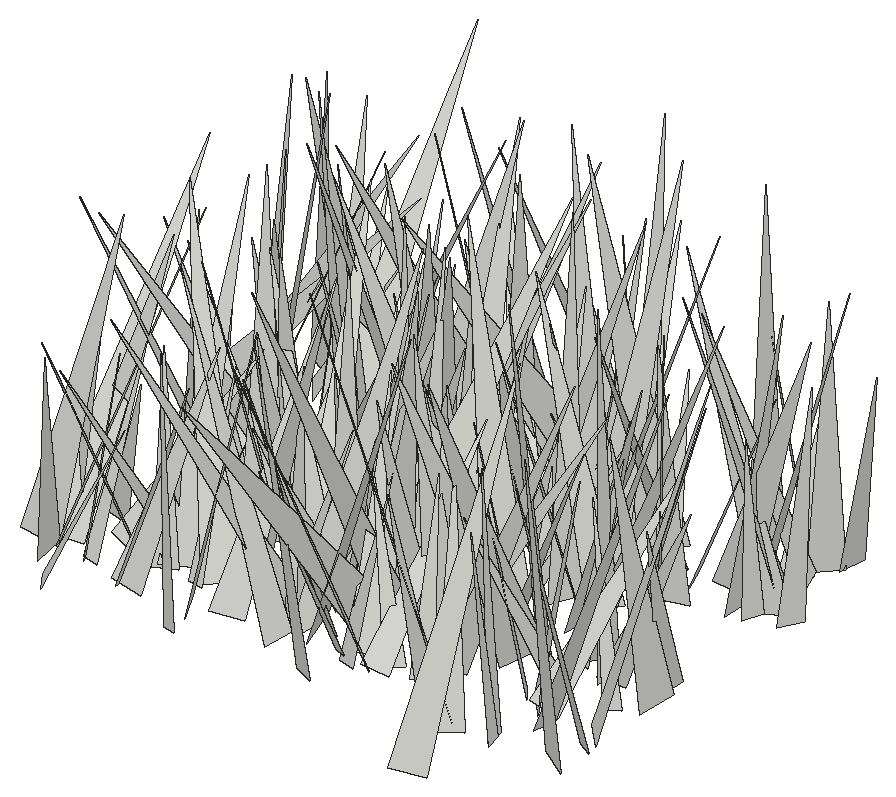
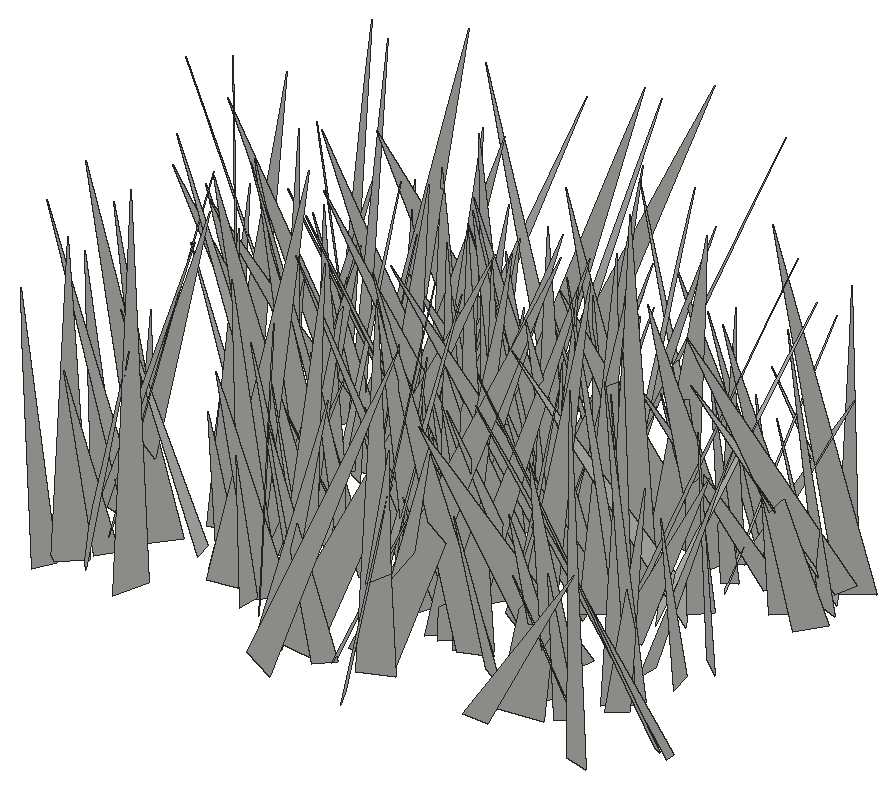
# SketchUp Ruby script. Lengths in inches.
U = 1.inch
M = Sketchup.active_model
def pt(a) = Geom::Point3d.new(a.map { |v| v * U })
def face(e, loops, mat)
  f = e.add_face(loops[0].map { |a| pt(a) })
  loops[1..].each { |l| e.add_face(l.map { |a| pt(a) }).erase! }
  f.material = f.back_material = mat if mat
  f
end
# faces: each face lists its corners as indices into pts; further lists are holes
def faces(e, pts, list, mat = nil) = list.each { |f| face(e, (f[0].is_a?(Array) ? f : [f]).map { |l| l.map { |i| pts[i] } }, mat) }
# xy, xz, yz: faces in a plane at the given z, y or x. An outline is a flat list of corners, or four numbers for a rectangle; further outlines are holes
def ring(l) = l.size == 4 ? [[l[0], l[1]], [l[2], l[1]], [l[2], l[3]], [l[0], l[3]]] : l.each_slice(2).to_a
def flat(e, list, mat, &to3) = list.each { |f| face(e, (f[0].is_a?(Array) ? f : [f]).map { |l| ring(l).map { |u, v| to3.(u, v) } }, mat) }
def xy(e, z, list, mat = nil) = flat(e, list, mat) { |x, y| [x, y, z] }
def xz(e, y, list, mat = nil) = flat(e, list, mat) { |x, z| [x, y, z] }
def yz(e, x, list, mat = nil) = flat(e, list, mat) { |y, z| [x, y, z] }
def lines(e, pts, list) = list.each { |a, b| e.add_line(pt(pts[a]), pt(pts[b])) }
# prism: a flat outline (further loops are holes) pulled along v
def prism(e, loops, v, mat = nil)
  f = face(e, loops, mat); d = Geom::Vector3d.new(v.map { |x| x * U })
  f.pushpull(f.normal.samedirection?(d) ? d.length : -d.length)
end
def box(e, o, s, mat = nil) = prism(e, [[o, [o[0] + s[0], o[1], o[2]], [o[0] + s[0], o[1] + s[1], o[2]], [o[0], o[1] + s[1], o[2]]]], [0, 0, s[2]], mat)
def at(x, y, z, deg = 0) = Geom::Transformation.translation(pt([x, y, z])) * Geom::Transformation.rotation(ORIGIN, Z_AXIS, deg.degrees)
def axes(o, x, y, z) = Geom::Transformation.new([*x, 0, *y, 0, *z, 0, *pt(o).to_a, 1])
def part(name) = M.definitions.add(name)
# library, detail: a bought-in or finely detailed component or shape, given as its bounding box
def library(name, o, s) = part(name).tap { |d| box(d.entities, o, s) }
def detail(e, o, s) = box(e.add_group.entities, o, s)
def put(e, d, t, mat = nil) = e.add_instance(d, t).tap { |i| i.material = mat if mat }
def group(e, t, mat = nil) = e.add_group.tap { |g| g.transformation = t; g.material = mat if mat }.entities
root = M.entities
c1 = part("fur_instance\#9")
p = [[0.8125,0,1.79],[0.67,-0.02,1.48],[0,-0.11,0],[0,0.11,0]]
faces(c1.entities,p,[[0,1,2,3]])
put(root,c1,axes([148.02,329.95,-27.1],[5.96387,-5.74764,0.45925],[-4.68382,-5.21453,-4.43673],[-3.36276,-2.93042,6.99418]))
put(root,c1,axes([148.79,327.89,-27.1],[-4.50054,-5.78959,0.45114],[-5.68851,4.51005,1.13049],[1.1678,-0.3432,7.24542]))
put(root,c1,axes([158.65,326.23,-27.1],[-3.10043,-5.65859,2.0595],[-5.81568,3.41455,0.62657],[1.56175,1.48157,6.42182]))
put(root,c1,axes([135.31,326.98,-27.1],[5.21183,-0.69159,1.00189],[-0.40075,-5.13378,-1.45906],[-1.14955,-1.3458,5.051]))
put(root,c1,axes([136.49,325.125,-27.1],[3.11612,2.14822,0.04863],[2.13222,-3.08072,-0.53874],[0.26618,-0.47091,3.74631]))
put(root,c1,axes([147.85,325.66,-27.1],[-3.61019,-4.99925,2.09321],[-5.40705,3.49453,-0.97958],[0.37125,2.28107,6.08822]))
put(root,c1,axes([144.81,329.15,-27.1],[-6.99156,-3.62516,0.34789],[-3.32905,6.6672,2.57109],[1.47657,-2.13338,7.444]))
put(root,c1,axes([156.08,326.05,-27.1],[-3.70453,-1.18645,1.17686],[-1.32576,3.8289,-0.31316],[1.01735,0.66938,3.87726]))
put(root,c1,axes([155.12,322.41,-27.1],[-6.41092,4.00729,0.82453],[3.32918,6.00061,-3.27831],[2.37798,2.40258,6.81256]))
put(root,c1,axes([154.44,325.61,-27.1],[-3.13208,3.88614,1.48189],[4.03166,3.29255,-0.11327],[1.02167,-1.07935,4.98991]))
put(root,c1,axes([142.17,325.18,-27.1],[2.11114,4.26728,1.69749],[4.08085,-2.60007,1.46097],[-2.10662,-0.76029,4.53125]))
put(root,c1,axes([152.23,327.2,-27.1],[0.17037,-4.40384,1.04145],[-4.5148,-0.2364,-0.26107],[-0.30825,1.02847,4.3994]))
put(root,c1,axes([153.88,326.43,-27.1],[-6.31099,-5.2237,1.0112],[-5.28027,5.95593,-2.18722],[-0.65451,2.31907,7.89505]))
put(root,c1,axes([141.64,327,-27.1],[5.91305,2.63208,1.30513],[2.84881,-5.85376,-1.10147],[-0.71801,-1.54954,6.37799]))
put(root,c1,axes([155.93,326.29,-27.1],[-4.75488,-0.89522,1.48594],[-1.16705,4.85843,-0.80746],[1.28353,1.10117,4.77057]))
put(root,c1,axes([147.875,327.68,-27.1],[-2.11494,-3.26023,0.3236],[-3.25153,2.04149,-0.68318],[-0.40176,0.64034,3.82562]))
put(root,c1,axes([138.71,326.98,-27.1],[4.6292,0.17151,0.50537],[0.17521,-4.6565,-0.02456],[-0.5041,-0.0434,4.63231]))
put(root,c1,axes([139.07,326.66,-27.1],[-0.2633,5.21725,2.01289],[5.21535,0.95622,-1.79623],[2.01778,-1.79073,4.90536]))
put(root,c1,axes([158.91,327.67,-27.1],[-3.27995,-3.84872,1.10692],[-4.00472,3.15616,-0.89264],[0.01123,1.42196,4.97734]))
put(root,c1,axes([146.15,328.58,-27.1],[7.97506,1.59703,0.67128],[1.71117,-7.75527,-1.87893],[-0.27022,-1.97686,7.91339]))
put(root,c1,axes([145.59,327.06,-27.1],[-7.05219,-0.0174,0.36445],[-0.04272,7.04446,-0.49029],[0.36236,0.49184,7.03515]))
put(root,c1,axes([138.22,330.29,-27.1],[-4.13321,-3.41194,0.20507],[-3.07913,3.85633,2.10107],[1.48403,-1.5014,4.93054]))
put(root,c1,axes([148.3125,330.61,-27.1],[0.33917,-8.30019,0.61155],[-8.21231,-0.43312,-1.32383],[-1.35096,0.54903,8.20095]))
put(root,c1,axes([138.89,328.01,-27.1],[-3.23089,-3.2407,0.20186],[-3.09319,2.98531,-1.58167],[-0.98745,1.25194,4.29408]))
put(root,c1,axes([134.44,327.56,-27.1],[1.86303,-6.4471,2.90273],[-6.99316,-1.23765,1.73947],[1.04242,3.21946,6.48153]))
put(root,c1,axes([146.71,328.67,-27.1],[-2.94659,-4.28728,0.79485],[-4.35538,2.84813,-0.78348],[-0.2081,1.09651,5.14289]))
put(root,c1,axes([153.12,331.42,-27.1],[6.488,-4.94571,0.82766],[-4.48999,-6.33233,-2.64212],[-2.23271,-1.63731,7.71838]))
put(root,c1,axes([150.02,328.08,-27.1],[-1.79664,3.17113,0.9039],[3.29721,1.71578,0.53432],[-0.03822,-1.04932,3.60534]))
put(root,c1,axes([136.61,327.37,-27.1],[2.93854,2.24557,1.05284],[2.03507,-3.11619,0.96641],[-1.41759,0.18132,3.56983]))
put(root,c1,axes([155.54,329.18,-27.1],[4.29125,3.34973,1.68987],[3.74545,-3.97458,-1.63261],[-0.21889,-2.33948,5.19327]))
put(root,c1,axes([145.97,328.53,-27.1],[-4.77809,0.40303,0.49366],[0.4272,4.79644,0.21897],[0.47289,-0.2608,4.79006]))
put(root,c1,axes([145.02,328.125,-27.1],[2.48119,3.58815,0.88423],[3.68479,-2.32113,-0.92071],[0.2811,-1.24521,4.2642]))
put(root,c1,axes([151.32,327.98,-27.1],[-2.54986,2.80817,1.27437],[2.87177,2.76487,-0.34653],[1.12374,-0.69377,3.77724]))
put(root,c1,axes([146.04,330.48,-27.1],[2.95419,-3.46444,1.08183],[-2.95275,-3.10527,-1.88109],[-2.11044,-0.50488,4.14621]))
put(root,c1,axes([139.31,328.55,-27.1],[1.67153,-3.68103,1.97281],[-4.08391,-1.88531,-0.05752],[-0.87388,1.76964,4.04237]))
put(root,c1,axes([136.89,327.36,-27.1],[1.45638,3.8911,0.37542],[3.87774,-1.48869,0.38679],[-0.49475,-0.21394,4.13668]))
put(root,c1,axes([154.88,330.97,-27.1],[-4.05266,-1.43323,0.72397],[-1.06557,3.87082,1.69814],[1.20119,-1.40176,3.94899]))
put(root,c1,axes([154.86,329.47,-27.1],[-3.48684,-2.54111,1.02639],[-2.66037,3.53733,-0.28017],[0.65812,0.83597,4.30544]))
put(root,c1,axes([134.55,329.12,-27.1],[2.41252,4.65389,1.89869],[5.02303,-2.30836,-0.72433],[-0.1815,-2.02404,5.19175]))
put(root,c1,axes([138.44,329.71,-27.1],[0.50859,-3.54434,0.97529],[-3.61365,-0.30136,0.78924],[0.67458,1.05784,3.49258]))
put(root,c1,axes([148.54,328.14,-27.1],[-2.22109,4.73282,1.14399],[4.81333,2.32397,-0.26934],[0.73496,-0.91711,5.22114]))
put(root,c1,axes([150.7,330.1875,-27.1],[3.54462,-5.56954,2.15269],[-5.7416,-3.86654,-0.54956],[-1.63946,1.49942,6.57891]))
put(root,c1,axes([135.71,330.37,-27.1],[0.50493,-3.90237,0.56248],[-3.75126,-0.30094,1.27958],[1.21364,0.69337,3.72104]))
put(root,c1,axes([149.64,327.45,-27.1],[-1.38897,4.86037,0.26759],[4.61521,1.40338,-1.53442],[1.54748,0.17706,4.81643]))
put(root,c1,axes([142.125,329.85,-27.1],[6.74375,-1.56753,0.95704],[-1.61805,-6.79399,0.27364],[-0.86892,0.48558,6.91813]))
put(root,c1,axes([140.84,328.32,-27.1],[1.32341,3.79294,0.4756],[3.74321,-1.38791,0.65276],[-0.77522,-0.22654,3.9638]))
put(root,c1,axes([142.03,331.95,-27.1],[-4.79038,-5.44103,1.36632],[-5.2062,4.98101,1.5825],[2.08977,-0.06337,7.07448]))
put(root,c1,axes([151.85,328.84,-27.1],[6.12264,-2.56902,1.18593],[-2.80714,-5.86992,1.77677],[-0.35534,2.10644,6.39763]))
put(root,c1,axes([151.7,332.15,-27.1],[4.33462,-5.23656,1.50263],[-4.77333,-4.57611,-2.17783],[-2.62578,-0.3257,6.43953]))
put(root,c1,axes([156.78,328.09,-27.1],[6.71372,1.26121,1.18447],[0.98901,-6.69183,1.51954],[-1.41968,1.3025,6.66001]))
put(root,c1,axes([148.57,327.17,-27.1],[3.46655,5.88623,0.70358],[5.62008,-3.5225,1.77941],[-1.8861,0.32244,6.59533]))
put(root,c1,axes([144,329.98,-27.1],[0.99186,4.25892,2.03749],[4.71935,-0.95274,-0.30591],[-0.13232,-2.05608,4.36218]))
put(root,c1,axes([141.59,329.05,-27.1],[-4.74257,5.72398,1.5327],[5.90767,4.72004,0.65254],[0.46105,-1.60076,7.40474]))
put(root,c1,axes([158.94,331.71,-27.1],[5.89812,-2.41371,1.85981],[-1.99813,-6.12286,-1.60962],[-2.30052,-0.87028,6.16628]))
put(root,c1,axes([158.6,328.57,-27.1],[5.3088,5.05785,1.00754],[5.10033,-5.36326,0.04959],[-0.76398,-0.65873,7.33231]))
put(root,c1,axes([143.11,327.25,-27.1],[-4.70627,4.28235,1.06672],[3.70191,4.67966,-2.45399],[2.40255,1.178,5.87073]))
put(root,c1,axes([148.3,331.74,-27.1],[-4.48343,0.78051,2.64752],[1.64873,4.80743,1.37477],[2.21365,-1.99978,4.33824]))
put(root,c1,axes([153.71,331.91,-27.1],[-3.953,-6.85404,2.35159],[-6.87911,4.39144,1.23577],[2.27722,1.36799,7.81517]))
put(root,c1,axes([136.97,329.07,-27.1],[0.32449,4.79651,0.65441],[4.29347,0.01783,-2.25961],[2.23626,-0.73022,4.24334]))
put(root,c1,axes([156.02,328.96,-27.1],[-0.77489,5.32124,0.74593],[4.8544,1.01638,-2.20776],[2.30365,-0.35187,4.90325]))
put(root,c1,axes([137.87,332.07,-27.1],[2.72527,-3.47225,0.02549],[-3.46346,-2.7159,0.33551],[0.24824,0.22715,4.40125]))
put(root,c1,axes([144.92,331.54,-27.1],[3.71508,-1.29272,0.27873],[-1.28155,-3.72443,-0.19222],[-0.32626,-0.0905,3.92887]))
put(root,c1,axes([134.17,330.49,-27.1],[3.16186,-4.77933,2.12939],[-5.21892,-2.70344,1.68164],[0.37303,2.68757,5.47827]))
put(root,c1,axes([135.22,327.62,-27.1],[5.40862,3.75774,0.29196],[3.28966,-4.95573,2.84217],[-1.83956,2.18614,5.94103]))
put(root,c1,axes([158.61,332.875,-27.1],[4.29129,-1.7599,0.57931],[-1.53313,-4.1935,-1.38278],[-1.04037,-1.07949,4.42723]))
put(root,c1,axes([157.96,330.41,-27.1],[-0.43735,3.78387,0.74816],[3.7266,0.2203,1.06426],[-0.99494,-0.83814,3.65736]))
put(root,c1,axes([145.99,332.95,-27.1],[2.29516,-7.21123,1.1617],[-7.23425,-2.07612,1.40519],[1.00849,1.5189,7.43607]))
put(root,c1,axes([139.01,333.09,-27.1],[-5.75391,-4.14909,0.07824],[-4.14913,5.75437,0.02082],[0.07564,0.02888,7.0938]))
put(root,c1,axes([156.68,331.96,-27.1],[2.75762,-4.13306,0.47465],[-3.98702,-2.46295,1.71739],[1.18791,1.32801,4.66232]))
put(root,c1,axes([139.53,328.97,-27.1],[-5.90287,3.96424,1.22936],[3.5461,5.92766,-2.08769],[2.15678,1.10365,6.7971]))
put(root,c1,axes([150.24,331.18,-27.1],[4.10846,4.74791,0.21399],[4.46685,-3.7608,-2.31765],[1.62348,-1.66782,5.83529]))
put(root,c1,axes([151.82,332.21,-27.1],[5.27208,0.02621,0.0042],[0.02652,-5.23568,-0.61848],[-0.0011,-0.61849,5.23574]))
put(root,c1,axes([135.03,328.06,-27.1],[-5.0261,5.87636,0.71878],[5.2638,4.86732,-2.98524],[2.70938,1.44485,7.13314]))
put(root,c1,axes([141.4,333.24,-27.1],[2.7716,-4.32676,0.73791],[-4.29866,-2.85215,-0.57784],[-0.88707,0.30254,5.10575]))
put(root,c1,axes([144.55,332.15,-27.1],[-1.98157,5.41612,3.08152],[6.10168,2.34277,-0.19399],[1.26474,-2.81671,5.76397]))
put(root,c1,axes([144.51,330.91,-27.1],[0.16131,6.95669,2.04491],[7.08472,0.28432,-1.5261],[1.54396,-2.03146,6.78915]))
put(root,c1,axes([146.39,331.33,-27.1],[-1.99924,6.11191,2.2816],[6.3463,2.375,-0.80119],[1.51181,-1.88733,6.38047]))
put(root,c1,axes([140.8,332.15,-27.1],[5.17413,-4.7343,3.23528],[-5.24163,-5.67192,0.08293],[-2.32507,2.25121,7.01272]))
put(root,c1,axes([143.2,332.24,-27.1],[-4.86777,3.35697,1.6535],[3.6105,4.92638,0.62739],[0.98366,-1.46972,5.8797]))
put(root,c1,axes([138.49,336.52,-27.1],[-6.95908,-3.88864,0.42907],[-3.38575,6.42493,3.31533],[1.96017,-2.70799,7.24975]))
put(root,c1,axes([156.37,332.2,-27.1],[-6.67663,-0.80436,2.4344],[-1.05353,7.05179,-0.55944],[2.33738,0.88086,6.7016]))
put(root,c1,axes([157.5,333.56,-27.1],[6.08028,3.66314,2.96745],[4.34842,-6.22849,-1.22118],[-1.82087,-2.64225,6.99265]))
put(root,c1,axes([140.65,334.31,-27.1],[4.51111,-4.76568,1.07484],[-4.75985,-4.61702,-0.49408],[-1.1004,0.43419,6.54353]))
put(root,c1,axes([154.84,332.49,-27.1],[2.00613,4.44684,1.43472],[4.67253,-1.91449,-0.59961],[-0.01581,-1.5549,4.84142]))
put(root,c1,axes([143.24,333.75,-27.1],[3.93197,-0.07434,1.3447],[0.21137,-4.06439,-0.84276],[-1.33006,-0.86567,3.84131]))
put(root,c1,axes([151.16,333.48,-27.1],[-2.98198,-2.20876,0.85448],[-2.34628,2.94214,-0.58291],[0.32208,0.98295,3.66484]))
put(root,c1,axes([153.21,334.51,-27.1],[6.29896,-1.22347,0.37639],[-1.1888,-6.29213,-0.55798],[-0.47466,-0.47719,6.39237]))
put(root,c1,axes([146.99,332.33,-27.1],[-6.72767,0.28008,1.7782],[-0.11729,6.79671,-1.51427],[1.7963,1.49276,6.56102]))
put(root,c1,axes([143.32,332.86,-27.1],[3.71678,-0.58843,1.31141],[-0.99782,-3.67326,1.17982],[-1.0346,1.42876,3.57333]))
put(root,c1,axes([151.24,336.56,-27.1],[-4.09949,-5.26965,1.04192],[-4.89422,4.20438,2.00758],[2.21389,-0.46331,6.36747]))
put(root,c1,axes([147.98,332.1,-27.1],[-6.09704,1.94582,1.05535],[1.61207,6.02238,-1.79053],[1.51697,1.42075,6.14444]))
put(root,c1,axes([147.14,334.9,-27.1],[-3.57828,-1.18752,0.86435],[-1.11493,3.67791,0.43741],[0.95617,-0.15551,3.74473]))
put(root,c1,axes([150.1,334.34,-27.1],[-5.03128,5.10175,2.45438],[5.52933,5.13327,0.66454],[1.21582,-2.23324,7.13442]))
put(root,c1,axes([155.03,332.48,-27.1],[6.92746,0.46404,1.30725],[0.06508,-6.75935,2.05449],[-1.38564,2.00246,6.63205]))
put(root,c1,axes([142.92,332.62,-27.1],[-3.90742,5.66938,0.63215],[5.60395,3.95813,-0.85923],[1.06639,-0.02677,6.83166]))
put(root,c1,axes([146.64,336.6,-27.1],[1.6071,-3.85332,0.26864],[-3.82652,-1.62792,-0.45895],[-0.52725,0.06941,4.14972]))
put(root,c1,axes([146.08,332.85,-27.1],[0.28527,8.21503,1.11931],[7.94931,0.04717,-2.37217],[2.35543,-1.15413,7.87026]))
put(root,c1,axes([146.5625,336.55,-27.1],[1.94153,-7.03493,2.68991],[-6.84514,-2.80689,-2.40016],[-3.14163,1.7682,6.89195]))
put(root,c1,axes([135.17,334.86,-27.1],[2.79154,3.79561,1.789],[3.98615,-3.06992,0.29332],[-1.31064,-1.25251,4.70248]))
put(root,c1,axes([138.73,335.11,-27.1],[-2.74524,3.88345,0.46197],[3.73915,2.44095,1.70042],[-1.14601,-1.33847,4.4414]))
put(root,c1,axes([149.73,335.05,-27.1],[1.87721,3.55983,2.07479],[3.45548,-2.60202,1.33802],[-2.2443,-1.02868,3.79553]))
put(root,c1,axes([155.05,335.29,-27.1],[4.65489,2.00226,0.76997],[2.06003,-4.68544,-0.26978],[-0.59848,-0.55448,5.06006]))
put(root,c1,axes([138.39,332.14,-27.1],[6.17595,4.1917,0.11311],[3.92557,-5.85042,2.46738],[-1.47413,1.98185,7.04448]))
put(root,c1,axes([145.65,335.82,-27.1],[-2.59622,-3.87524,1.56211],[-4.17566,2.47102,-0.8099],[0.14666,1.75346,4.59368]))
put(root,c1,axes([136.68,336.55,-27.1],[-4.93591,-0.64757,0.62999],[-0.58328,4.95621,0.52453],[0.68994,-0.44273,4.95049]))
put(root,c1,axes([142.77,335.02,-27.1],[4.39475,-2.24157,1.41228],[-2.61052,-4.13054,1.56743],[-0.4521,2.06082,4.67778]))
put(root,c1,axes([146.18,336.84,-27.1],[2.32734,-2.83374,0.7234],[-2.82694,-2.41664,-0.37171],[-0.74954,0.31569,3.64807]))
put(root,c1,axes([153.16,336.07,-27.1],[1.40362,-5.52471,3.15038],[-5.88186,-2.35471,-1.50878],[-2.41887,2.51999,5.49692]))
put(root,c1,axes([142.69,336.65,-27.1],[-2.18314,-4.32344,1.23175],[-4.48368,1.99494,-0.94459],[-0.32548,1.51774,4.75036]))
put(root,c1,axes([151.72,335.61,-27.1],[-6.82221,1.72842,2.33339],[1.55801,7.20655,-0.7829],[2.45045,0.23004,6.99407]))
put(root,c1,axes([150.13,336.11,-27.1],[2.36408,2.77163,0.06713],[2.67068,-2.25294,-1.03299],[0.74428,-0.71945,3.49339]))
put(root,c1,axes([143.6875,338.3,-27.1],[-2.92587,-7.18113,1.16279],[-7.26033,2.80394,-0.95233],[-0.45638,1.43204,7.69561]))
put(root,c1,axes([144.07,334.52,-27.1],[-6.55777,-1.69063,0.96933],[-1.94723,5.82112,-3.02077],[0.07829,3.17151,6.06115]))
put(root,c1,axes([143.35,338.85,-27.1],[6.03142,-3.81553,0.06105],[-3.78285,-5.99326,-0.84318],[-0.50203,-0.68018,7.08699]))
put(root,c1,axes([141.83,335.84,-27.1],[3.01287,6.59159,3.14785],[6.68601,-3.85992,1.68335],[-2.94198,-2.02171,7.04931]))
put(root,c1,axes([141.3,333.76,-27.1],[8.13391,1.72844,0.70897],[1.41113,-7.75982,2.72846],[-1.22428,2.53935,7.85515]))
put(root,c1,axes([144.98,334.99,-27.1],[4.52009,6.67395,0.30614],[6.59904,-4.40227,-1.46264],[1.04307,-1.07006,7.92676]))
put(root,c1,axes([142.47,339.125,-27.1],[1.32188,-7.44707,0.58602],[-7.30684,-1.16527,1.67389],[1.55318,0.85612,7.37593]))
put(root,c1,axes([136.04,339.01,-27.1],[5.72206,-2.67718,0.30846],[-2.55509,-5.6197,-1.37653],[-0.85672,-1.12072,6.16558]))
put(root,c1,axes([154.79,337.8125,-27.1],[1.69924,-5.28596,1.58911],[-5.50046,-1.7602,0.02657],[-0.46001,1.5213,5.5523]))
put(root,c1,axes([135.3,336.42,-27.1],[-3.53887,0.08812,1.47041],[-0.2173,3.75324,-0.74791],[1.45693,0.77383,3.46005]))
put(root,c1,axes([150.95,338.52,-27.1],[-1.08369,-5.40972,1.03151],[-5.49173,1.14023,0.21038],[0.41232,0.96864,5.51318]))
put(root,c1,axes([137.13,337,-27.1],[6.97385,3.06548,2.09729],[3.25235,-7.19468,-0.2986],[-1.79388,-1.12684,7.61201]))
put(root,c1,axes([152.11,338.59,-27.1],[-3.71284,-0.24914,0.82183],[0.046,3.58403,1.29433],[0.85753,-1.27095,3.48884]))
put(root,c1,axes([137.36,336.57,-27.1],[3.68214,4.39884,2.0354],[4.4735,-4.06815,0.69917],[-1.86561,-1.07294,5.69378]))
put(root,c1,axes([143.95,338.87,-27.1],[-6.33507,2.2676,3.27677],[3.13305,6.63723,1.4641],[2.46237,-2.61105,6.56746]))
put(root,c1,axes([152.89,340.33,-27.1],[-1.67702,-6.45132,0.05531],[-6.32349,1.655,1.30744],[1.27907,-0.27646,6.53625]))
put(root,c1,axes([142.98,338.3,-27.1],[2.13927,-3.81253,0.27989],[-3.71667,-1.99926,1.17453],[0.89447,0.81104,4.21098]))
put(root,c1,axes([146.87,339.23,-27.1],[2.00782,-4.43373,0.05819],[-4.43409,-2.00742,0.0429],[0.01508,0.0707,4.86698]))
put(root,c1,axes([148.5,337.56,-27.1],[4.58596,6.39713,1.96066],[6.63658,-4.04695,-2.31874],[0.85046,-2.91504,7.52182]))
put(root,c1,axes([144.14,336.14,-27.1],[-3.10832,3.75001,0.92239],[3.63037,3.24121,-0.94342],[1.31674,-0.08395,4.77852]))
put(root,c1,axes([141.85,336.15,-27.1],[4.95008,1.27612,1.12304],[0.89586,-4.89693,1.61571],[-1.4447,1.33589,4.84988]))
put(root,c1,axes([151.08,337.77,-27.1],[7.89024,2.57718,0.73013],[2.64489,-7.85516,-0.85554],[-0.42369,-1.04189,8.25626]))
put(root,c1,axes([145.67,337.09,-27.1],[1.56469,4.5597,1.40699],[4.65343,-1.78584,0.61247],[-1.05645,-1.11294,4.78163]))
put(root,c1,axes([150,336.64,-27.1],[0.07202,5.27236,0.64208],[5.29211,-0.12578,0.43929],[-0.45123,-0.63374,5.25452]))
put(root,c1,axes([157.63,338.74,-27.1],[3.35457,-1.66316,1.27005],[-1.64462,-3.57909,-0.343],[-1.29397,0.23728,3.72849]))
put(root,c1,axes([146.74,337.125,-27.1],[-4.01234,0.85775,1.7856],[0.34464,4.27421,-1.27879],[1.95072,1.00913,3.89863]))
put(root,c1,axes([157.84,340.3125,-27.1],[-5.81163,-3.8947,1.27527],[-3.71182,5.94036,1.22659],[1.73708,-0.33677,6.88761]))
put(root,c1,axes([135.78,339.38,-27.1],[3.23004,-2.47849,1.2151],[-2.38486,-3.44753,-0.69249],[-1.3899,0.15559,4.01205]))
put(root,c1,axes([144.87,341.88,-27.1],[1.87232,-8.06563,0.81969],[-7.60481,-2.03883,-2.69107],[-2.80947,0.14362,7.83059]))
put(root,c1,axes([155.875,339.8,-27.1],[2.64878,-6.42579,1.07864],[-6.29914,-2.22772,2.19734],[1.66585,1.79353,6.59382]))
put(root,c1,axes([146.05,339.2,-27.1],[4.40996,1.53054,2.75088],[1.88618,-5.07543,-0.19988],[-2.52036,-1.1203,4.66373]))
put(root,c1,axes([151.84,337.22,-27.1],[6.54564,-3.57049,3.76512],[-4.66006,-6.71077,1.73761],[-2.28219,3.46223,7.25083]))
put(root,c1,axes([156.87,338.81,-27.1],[6.13024,0.22864,1.74835],[0.20896,-6.37456,0.10097],[-1.75081,0.03976,6.13367]))
put(root,c1,axes([136.17,337.83,-27.1],[2.58836,6.22661,1.98748],[6.38761,-2.86286,0.6503],[-1.38536,-1.56644,6.71174]))
put(root,c1,axes([147.49,343.02,-27.1],[4.76692,-6.38187,0.99404],[-5.33821,-4.5884,-3.85875],[-3.63592,-1.6304,6.96863]))
put(root,c1,axes([159.02,339.13,-27.1],[4.44334,-1.86269,1.64457],[-2.02269,-4.66849,0.17731],[-1.44323,0.80817,4.81471]))
put(root,c1,axes([146.85,339.35,-27.1],[-5.72763,-4.55632,1.57593],[-4.80185,5.61014,-1.23206],[0.43111,1.95337,7.21442]))
put(root,c1,axes([158.12,339.33,-27.1],[-0.65544,-6.57541,2.82853],[-6.91722,-0.14862,-1.94837],[-1.84083,2.89967,6.31422]))
put(root,c1,axes([144.26,338.19,-27.1],[3.571,6.90444,0.98118],[6.89309,-3.32732,-1.67343],[1.05801,-1.62595,7.59098]))
put(root,c1,axes([154.35,339.5,-27.1],[4.46845,1.48023,0.19389],[1.49287,-4.43008,-0.58427],[0.00126,-0.6156,4.67084]))
put(root,c1,axes([138.26,341.72,-27.1],[1.76512,-7.95634,1.31885],[-8.03843,-1.84494,-0.37166],[-0.65291,1.20466,8.14131]))
put(root,c1,axes([152.01,340.8,-27.1],[2.92408,-7.38877,2.72238],[-7.56214,-3.44459,-1.22649],[-2.19528,2.02396,7.85111]))
put(root,c1,axes([145.48,337.59,-27.1],[5.43527,-3.00495,4.38513],[-4.48513,-5.95873,1.47596],[-2.85354,3.64214,6.0327]))
put(root,c1,axes([142.23,339.31,-27.1],[0.54119,7.40359,2.44886],[7.61955,0.0202,-1.74498],[1.65906,-2.50787,7.21533]))
put(root,c1,axes([157.67,341.83,-27.1],[-5.8236,-1.97497,1.08531],[-1.72724,5.8434,1.36532],[1.44743,-0.9731,5.99589]))
put(root,c1,axes([150.25,339.33,-27.1],[-7.50799,1.69583,1.59774],[1.55933,7.66276,-0.80567],[1.73121,0.45255,7.65484]))
put(root,c1,axes([132.29,340.76,-27.1],[4.7067,5.43888,0.18038],[4.50837,-3.76361,-4.15655],[3.04771,-2.83211,5.87006]))
put(root,c1,axes([153.1,339.65,-27.1],[-2.61192,2.51011,0.78878],[2.46687,2.72278,-0.49597],[0.91509,-0.17543,3.58843]))
put(root,c1,axes([148.5,340.86,-27.1],[3.90059,1.73334,0.99556],[1.91928,-3.85762,-0.80331],[-0.55855,-1.15086,4.19211]))
put(root,c1,axes([156.875,340,-27.1],[6.30339,2.19635,1.13005],[2.22882,-6.39265,-0.00763],[-1.06457,-0.37914,6.67507]))
put(root,c1,axes([145.35,340.4,-27.1],[-4.286,2.05614,0.85108],[2.13965,4.31523,0.34994],[0.6115,-0.68765,4.74078]))
put(root,c1,axes([132.9375,340.68,-27.1],[5.32286,5.30667,0.20638],[4.93366,-4.8331,-2.97258],[1.96528,-2.23975,6.90343]))
put(root,c1,axes([138.51,339.5625,-27.1],[-1.52341,4.48001,0.30788],[4.47725,1.54034,-0.26007],[0.34571,-0.20714,4.72479]))
put(root,c1,axes([145.82,342.77,-27.1],[-3.34335,-1.51871,0.13226],[-1.40215,3.18862,1.16988],[0.59829,-1.01398,3.48078]))
put(root,c1,axes([149.73,339.79,-27.1],[1.82838,5.64567,1.15342],[5.69001,-1.95997,0.57384],[-0.90985,-0.91206,5.90655]))
put(root,c1,axes([144.09,342.6,-27.1],[1.85268,-6.56464,1.39244],[-6.70428,-1.74747,0.68181],[0.2934,1.52239,6.78691]))
put(root,c1,axes([150.32,341.38,-27.1],[-4.40906,-3.22075,2.19411],[-3.50304,4.72714,-0.10035],[1.70765,1.38134,5.45921]))
put(root,c1,axes([138.0625,339.61,-27.1],[-5.38629,2.97439,0.98855],[2.72826,5.41671,-1.43257],[1.54299,0.80541,5.98388]))
put(root,c1,axes([135.36,341.81,-27.1],[3.3764,2.66955,0.1135],[2.47122,-3.05035,-1.76859],[1.01611,-1.452,3.92412]))
put(root,c1,axes([136.83,341,-27.1],[-1.83169,3.1238,0.57494],[3.14275,1.87858,-0.19441],[0.4602,-0.39568,3.61599]))
put(root,c1,axes([140.72,340.19,-27.1],[1.48106,4.37962,0.44895],[4.22706,-1.54701,1.14671],[-1.23071,-0.04293,4.4788]))
put(root,c1,axes([157.58,342.9375,-27.1],[-3.8078,3.44308,3.43375],[4.19662,4.52997,0.11149],[2.45637,-2.40193,5.13242]))
put(root,c1,axes([134.57,343.21,-27.1],[-2.31612,-6.1908,2.36322],[-6.27799,2.85121,1.3163],[2.12077,1.67923,6.47748]))
put(root,c1,axes([143.94,344.63,-27.1],[-6.24986,-4.52728,1.84324],[-4.17742,6.50052,1.80193],[2.5383,-0.44892,7.504]))
put(root,c1,axes([150.4,340.58,-27.1],[-3.17134,4.85922,0.78552],[4.77597,3.26378,-0.90795],[1.19131,-0.14895,5.73106]))
put(root,c1,axes([145.62,340.79,-27.1],[-3.60755,4.52257,0.00535],[4.517,3.60276,0.29145],[-0.22451,-0.18592,5.77782]))
put(root,c1,axes([150.79,340.82,-27.1],[-7.20595,2.28011,2.02761],[1.9171,7.42879,-1.54068],[2.37378,0.922,7.39939]))
put(root,c1,axes([138.86,338.17,-27.1],[-6.04626,5.73242,0.3376],[5.11125,5.59588,-3.47751],[2.61721,2.31459,7.57131]))
put(root,c1,axes([156.89,341.79,-27.1],[-2.21972,3.26489,1.22418],[3.2229,2.47495,-0.75684],[1.3308,-0.54808,3.87477]))
put(root,c1,axes([154.65,343.21,-27.1],[7.21029,-1.27081,2.71678],[-1.16788,-7.70491,-0.50453],[-2.76259,-0.05954,7.30402]))
put(root,c1,axes([157.25,342.58,-27.1],[2.56501,3.25674,2.5986],[3.3721,-3.41499,0.95138],[-2.44704,-1.29222,4.03491]))
put(root,c1,axes([158.07,343.8,-27.1],[4.83385,-1.43847,0.54232],[-1.36908,-4.84202,-0.64023],[-0.69925,-0.46374,5.00254]))
put(root,c1,axes([148.16,343.64,-27.1],[-4.52682,2.09063,1.69581],[2.46981,4.54531,0.98938],[1.07078,-1.64562,4.88712]))
put(root,c1,axes([139.35,342.92,-27.1],[-2.95637,3.32548,0.26078],[3.10336,2.61427,1.84435],[-1.22309,-1.40488,4.04936]))
put(root,c1,axes([146,343.0625,-27.1],[1.71183,-4.04593,1.56999],[-4.29437,-1.33542,1.2409],[0.62675,1.9005,4.21427]))
put(root,c1,axes([147.77,344.62,-27.1],[-2.28095,-6.51713,0.89519],[-6.46928,2.05047,-1.55597],[-1.19279,1.34151,6.72716]))
